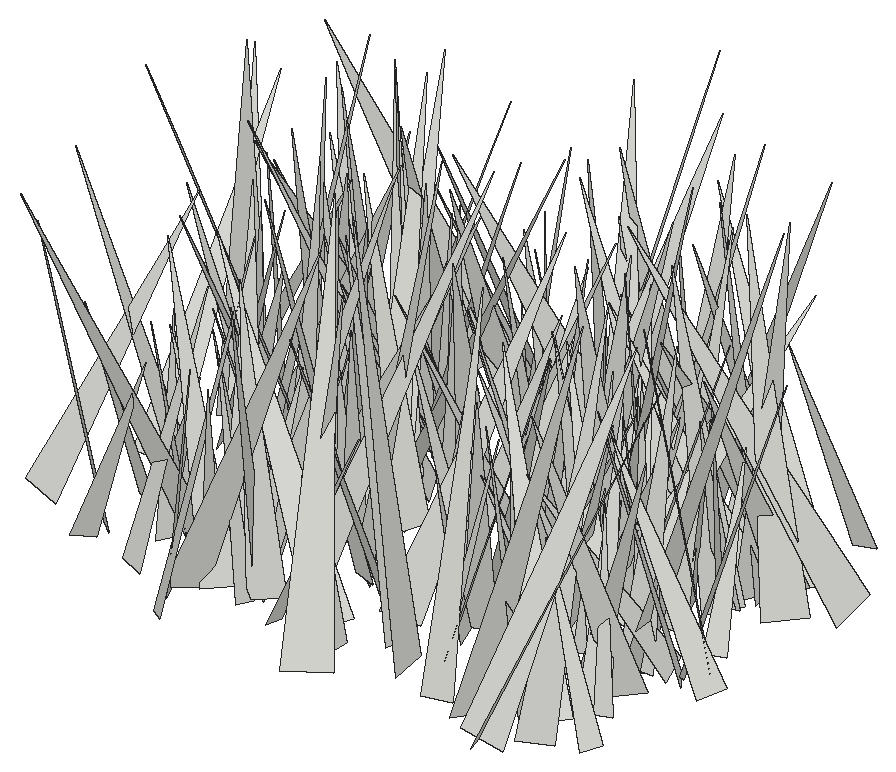
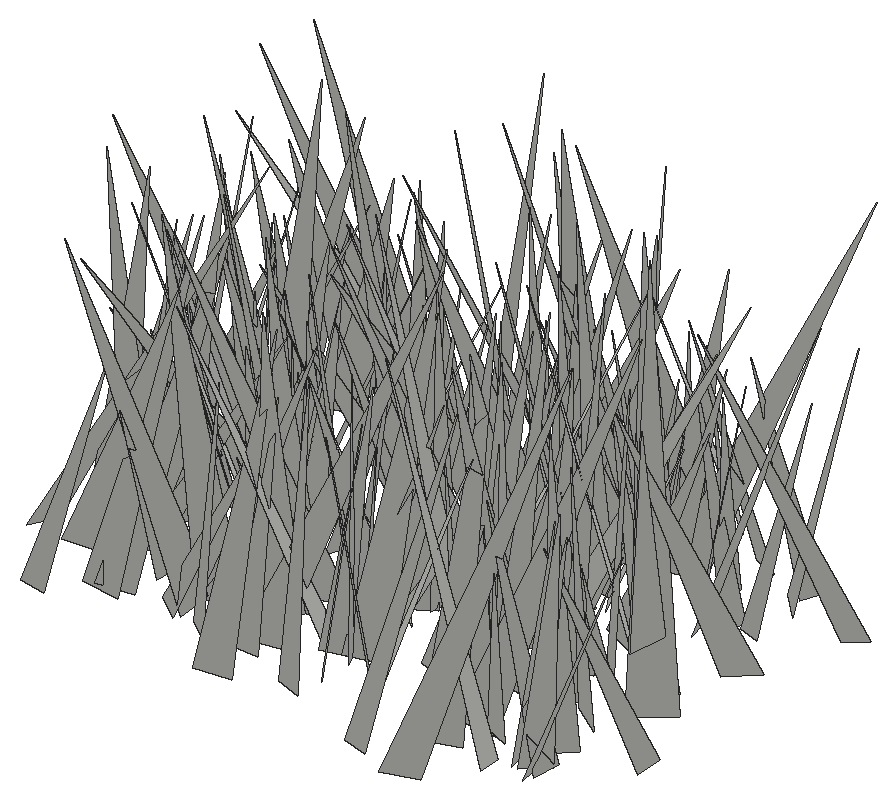
# SketchUp Ruby script. Lengths in inches.
U = 1.inch
M = Sketchup.active_model
def pt(a) = Geom::Point3d.new(a.map { |v| v * U })
def face(e, loops, mat)
  f = e.add_face(loops[0].map { |a| pt(a) })
  loops[1..].each { |l| e.add_face(l.map { |a| pt(a) }).erase! }
  f.material = f.back_material = mat if mat
  f
end
# faces: each face lists its corners as indices into pts; further lists are holes
def faces(e, pts, list, mat = nil) = list.each { |f| face(e, (f[0].is_a?(Array) ? f : [f]).map { |l| l.map { |i| pts[i] } }, mat) }
# xy, xz, yz: faces in a plane at the given z, y or x. An outline is a flat list of corners, or four numbers for a rectangle; further outlines are holes
def ring(l) = l.size == 4 ? [[l[0], l[1]], [l[2], l[1]], [l[2], l[3]], [l[0], l[3]]] : l.each_slice(2).to_a
def flat(e, list, mat, &to3) = list.each { |f| face(e, (f[0].is_a?(Array) ? f : [f]).map { |l| ring(l).map { |u, v| to3.(u, v) } }, mat) }
def xy(e, z, list, mat = nil) = flat(e, list, mat) { |x, y| [x, y, z] }
def xz(e, y, list, mat = nil) = flat(e, list, mat) { |x, z| [x, y, z] }
def yz(e, x, list, mat = nil) = flat(e, list, mat) { |y, z| [x, y, z] }
def lines(e, pts, list) = list.each { |a, b| e.add_line(pt(pts[a]), pt(pts[b])) }
# prism: a flat outline (further loops are holes) pulled along v
def prism(e, loops, v, mat = nil)
  f = face(e, loops, mat); d = Geom::Vector3d.new(v.map { |x| x * U })
  f.pushpull(f.normal.samedirection?(d) ? d.length : -d.length)
end
def box(e, o, s, mat = nil) = prism(e, [[o, [o[0] + s[0], o[1], o[2]], [o[0] + s[0], o[1] + s[1], o[2]], [o[0], o[1] + s[1], o[2]]]], [0, 0, s[2]], mat)
def at(x, y, z, deg = 0) = Geom::Transformation.translation(pt([x, y, z])) * Geom::Transformation.rotation(ORIGIN, Z_AXIS, deg.degrees)
def axes(o, x, y, z) = Geom::Transformation.new([*x, 0, *y, 0, *z, 0, *pt(o).to_a, 1])
def part(name) = M.definitions.add(name)
# library, detail: a bought-in or finely detailed component or shape, given as its bounding box
def library(name, o, s) = part(name).tap { |d| box(d.entities, o, s) }
def detail(e, o, s) = box(e.add_group.entities, o, s)
def put(e, d, t, mat = nil) = e.add_instance(d, t).tap { |i| i.material = mat if mat }
def group(e, t, mat = nil) = e.add_group.tap { |g| g.transformation = t; g.material = mat if mat }.entities
root = M.entities
c1 = part("fur_instance\#9")
p = [[0.8125,0,1.79],[0.67,-0.02,1.48],[0,-0.11,0],[0,0.11,0]]
faces(c1.entities,p,[[0,1,2,3]])
put(root,c1,axes([118.75,215.38,-27.1],[-3.28983,-1.54802,1.9149],[-2.00034,3.5437,-0.57187],[1.43591,1.38997,3.59058]))
put(root,c1,axes([118.43,218.14,-27.1],[-1.35129,-7.71927,0.81651],[-7.46816,1.06686,-2.27338],[-2.11671,1.16382,7.49966]))
put(root,c1,axes([125.51,216.04,-27.1],[-3.60239,-0.15597,0.87969],[-0.19043,3.7046,-0.12301],[0.87288,0.16452,3.60367]))
put(root,c1,axes([136.4,215.91,-27.1],[-3.21224,1.96871,0.46482],[2.01704,3.18335,0.45637],[0.15311,-0.63315,3.7398]))
put(root,c1,axes([120.625,217.96,-27.1],[5.99792,1.55177,2.60045],[2.40829,-5.94226,-2.00876],[-1.83589,-2.72525,5.86071]))
put(root,c1,axes([131.79,215.22,-27.1],[7.44072,-1.6859,2.03296],[-2.09272,-7.4711,1.46382],[-1.61112,1.91833,7.48758]))
put(root,c1,axes([133.125,214.13,-27.1],[-0.55252,7.61083,1.2014],[7.43516,0.84266,-1.91879],[2.02152,-1.01911,7.38568]))
put(root,c1,axes([134.1875,215.24,-27.1],[-5.16392,-1.1559,0.80889],[-1.35151,4.93357,-1.57791],[0.40477,1.72635,5.05098]))
put(root,c1,axes([125.68,214.08,-27.1],[-5.56313,6.05819,1.00831],[6.02083,5.64819,-0.71719],[1.2116,-0.25113,8.19364]))
put(root,c1,axes([114.08,216.65,-27.1],[3.45367,-2.54495,0.42724],[-2.57712,-3.36456,0.79082],[0.1334,0.88889,4.21654]))
put(root,c1,axes([123.74,216.53,-27.1],[6.28963,-0.96384,2.1084],[-1.07131,-6.61487,0.17192],[-2.05588,0.49827,6.36073]))
put(root,c1,axes([118.91,216.05,-27.1],[6.76451,-3.26106,1.25254],[-3.47694,-6.54929,1.72622],[-0.33809,2.1058,7.30844]))
put(root,c1,axes([128.125,216.47,-27.1],[-7.87878,-1.52664,2.20407],[-1.70967,8.13085,-0.47967],[2.06533,0.90687,8.01097]))
put(root,c1,axes([133.12,213.78,-27.1],[6.18332,3.30926,0.01495],[3.17233,-5.93637,1.96995],[-0.9422,1.73008,6.73082]))
put(root,c1,axes([122.71,216.04,-27.1],[3.9235,0.14114,0.37721],[0.06723,-3.8717,0.74932],[-0.3971,0.73898,3.85386]))
put(root,c1,axes([119.34,213.99,-27.1],[4.35483,5.04158,0.80125],[4.65214,-4.35304,2.10539],[-2.1017,0.81089,6.32055]))
put(root,c1,axes([118.79,217.6,-27.1],[3.85883,-1.0172,1.02296],[-0.87371,-3.97244,-0.65425],[-1.14794,-0.39587,3.93665]))
put(root,c1,axes([129.71,215.92,-27.1],[2.50571,3.8301,0.73521],[3.84486,-2.57244,0.29737],[-0.65369,-0.44905,4.56726]))
put(root,c1,axes([121.5625,217.11,-27.1],[-3.51075,4.42455,2.16586],[4.8357,3.60279,0.47842],[0.94002,-2.00904,5.62789]))
put(root,c1,axes([119.84,216.78,-27.1],[-3.34146,5.15286,1.47209],[5.35695,3.16362,1.08579],[-0.14849,-1.82317,6.0447]))
put(root,c1,axes([116.61,216.07,-27.1],[2.03381,4.83721,0.83738],[4.90479,-2.04045,-0.1258],[-0.20703,-0.82108,5.24587]))
put(root,c1,axes([121.15,216.45,-27.1],[-4.31173,0.11749,0.33288],[0.02447,4.16916,-1.1546],[0.35215,1.14887,4.15592]))
put(root,c1,axes([114.28,217.63,-27.1],[-4.01169,-3.78695,1.3287],[-4.00574,3.89344,-0.9976],[0.2459,1.64323,5.42581]))
put(root,c1,axes([125.25,219.08,-27.1],[-2.82637,-5.01502,0.69558],[-5.06125,2.81969,-0.23605],[0.13409,0.7222,5.75179]))
put(root,c1,axes([132.3,217.14,-27.1],[-3.8319,-0.08961,1.0116],[-0.27638,3.8917,-0.7022],[0.97723,0.7493,3.76807]))
put(root,c1,axes([134.18,216.58,-27.1],[-3.78417,5.30239,0.2634],[5.25954,3.70033,1.07214],[-0.72248,-0.83479,6.42541]))
put(root,c1,axes([124.35,217.11,-27.1],[-4.44973,5.42889,0.1833],[5.21151,4.19987,2.12315],[-1.53186,-1.48148,6.69068]))
put(root,c1,axes([135.0625,219.58,-27.1],[2.07945,-5.56592,1.40736],[-5.43571,-2.39045,-1.42237],[-1.84751,0.76846,5.76892]))
put(root,c1,axes([130.25,215.33,-27.1],[0.51601,7.02264,0.2402],[6.84431,-0.55684,1.57697],[-1.5908,-0.11784,6.86272]))
put(root,c1,axes([120.35,217.64,-27.1],[0.83525,-3.69964,2.10924],[-4.22949,-0.46947,0.8514],[0.49764,2.21949,3.69595]))
put(root,c1,axes([118.83,218.36,-27.1],[-2.76713,3.18046,1.2921],[3.43249,2.58898,0.97827],[0.05304,-1.61979,4.10065]))
put(root,c1,axes([134.68,215.03,-27.1],[-6.77077,3.15469,0.89527],[2.64884,6.47215,-2.77341],[1.93319,2.18084,6.93567]))
put(root,c1,axes([117.28,218.42,-27.1],[-3.57369,-1.9669,1.0397],[-2.0892,3.64317,-0.28897],[0.76478,0.76131,4.06896]))
put(root,c1,axes([128.33,219.27,-27.1],[-3.2792,-1.26365,1.37089],[-0.97388,3.52607,0.9207],[1.58988,-0.44645,3.3915]))
put(root,c1,axes([128.36,219.98,-27.1],[2.49567,-4.97649,0.70111],[-5.02561,-2.47346,0.33254],[-0.01412,0.77585,5.55727]))
put(root,c1,axes([120.59,217.56,-27.1],[4.03025,7.20792,1.49357],[7.34455,-3.82368,-1.36555],[0.49235,-1.96292,8.14446]))
put(root,c1,axes([126.84,217.54,-27.1],[-7.00273,-0.39667,0.95685],[-0.59042,6.90153,-1.45992],[0.85107,1.52402,6.86034]))
put(root,c1,axes([116.36,218.28,-27.1],[-3.76859,1.24193,1.36163],[1.17189,4.00702,-0.41131],[1.42236,-0.01087,3.94658]))
put(root,c1,axes([114.88,219.91,-27.1],[1.3305,-3.93215,0.09517],[-3.71952,-1.22514,1.38031],[1.27907,0.52755,3.91494]))
put(root,c1,axes([135.32,217.88,-27.1],[-0.19051,3.61425,0.52762],[3.57644,0.0773,0.76192],[-0.74175,-0.55561,3.53816]))
put(root,c1,axes([132.47,219.64,-27.1],[-4.25232,-1.15186,0.17503],[-1.13335,4.24309,0.38907],[0.27009,-0.33025,4.38835]))
put(root,c1,axes([114.16,219.99,-27.1],[-1.28236,-4.10189,0.60594],[-4.14572,1.27987,-0.10961],[0.07509,0.61118,4.29626]))
put(root,c1,axes([133.57,219.35,-27.1],[4.86131,-2.02952,0.59697],[-2.06386,-4.87843,0.22145],[-0.46454,0.43544,5.26329]))
put(root,c1,axes([119.67,218.16,-27.1],[-2.53684,6.34204,1.9532],[6.60869,2.60398,0.12835],[0.60133,-1.86275,6.82939]))
put(root,c1,axes([120.46,218.35,-27.1],[3.86814,-0.78573,1.02615],[-1.07279,-3.75781,1.16655],[-0.72076,1.37634,3.77081]))
put(root,c1,axes([135.16,221.83,-27.1],[-5.02387,-1.18033,0.42976],[-0.88594,4.58548,2.23734],[0.8905,-2.09699,4.65046]))
put(root,c1,axes([128.69,217.84,-27.1],[4.75922,3.00167,0.77273],[2.8511,-4.79497,1.06623],[-1.21588,0.50555,5.5248]))
put(root,c1,axes([128.02,220.89,-27.1],[6.9866,-0.46387,0.39437],[-0.38095,-6.874,-1.33651],[-0.47495,-1.31005,6.87325]))
put(root,c1,axes([111.05,218.15,-27.1],[0.65701,6.39206,0.99008],[6.12037,-0.29236,-2.17392],[2.09278,-1.15171,6.04683]))
put(root,c1,axes([134.65,218.26,-27.1],[-3.96377,3.38106,0.80717],[3.27975,4.04327,-0.83051],[1.15166,0.12228,5.14327]))
put(root,c1,axes([120.79,221.17,-27.1],[2.81621,-4.35059,0.38195],[-4.36621,-2.81499,0.12899],[-0.09891,0.39082,5.18093]))
put(root,c1,axes([123.21,220.25,-27.1],[-3.81075,-5.76969,1.72606],[-6.01138,3.52106,-1.50194],[-0.36316,2.25903,6.74947]))
put(root,c1,axes([115.74,220.55,-27.1],[-6.60705,-1.5953,0.55499],[-1.61141,6.62494,-0.14037],[0.50631,0.26714,6.79547]))
put(root,c1,axes([135.77,221.49,-27.1],[-4.16981,-3.31895,0.85743],[-3.36405,4.22145,-0.01946],[0.65859,0.54939,5.32938]))
put(root,c1,axes([122.56,217.82,-27.1],[3.274,7.7332,0.0389],[7.72076,-3.26624,-0.49451],[0.44025,-0.22856,8.38313]))
put(root,c1,axes([130.0625,219.08,-27.1],[4.92859,0.75105,0.39032],[0.57555,-4.66461,1.7081],[-0.62062,1.63853,4.68375]))
put(root,c1,axes([130.85,221.33,-27.1],[4.88822,-0.89007,0.63341],[-0.87396,-4.92864,-0.18113],[-0.65546,-0.06625,4.96529]))
put(root,c1,axes([137.24,221.32,-27.1],[-3.88127,2.88585,0.74535],[2.95869,3.58243,1.53633],[-0.36036,-1.66913,4.58608]))
put(root,c1,axes([117.11,221.5,-27.1],[-3.35519,-0.75879,1.11745],[-0.66434,3.53232,0.40387],[1.17606,-0.1694,3.41613]))
put(root,c1,axes([122.875,220.59,-27.1],[4.94057,6.27292,2.28459],[6.62263,-4.9638,-0.69253],[-0.84236,-2.23369,7.95482]))
put(root,c1,axes([121.28,222.14,-27.1],[4.3252,-1.84495,1.08949],[-1.74272,-4.45705,-0.62914],[-1.2465,-0.1704,4.65998]))
put(root,c1,axes([119.76,220.89,-27.1],[-1.17344,-6.36654,3.3674],[-7.15717,1.41187,0.17527],[0.80444,3.27459,6.4714]))
put(root,c1,axes([133.66,220.24,-27.1],[-3.54308,4.52564,0.44169],[4.5332,3.47169,0.79207],[-0.35583,-0.83417,5.69276]))
put(root,c1,axes([119.19,221.23,-27.1],[-3.56795,-1.90054,0.20659],[-1.88749,3.43261,-1.0196],[-0.30353,0.99505,3.91187]))
put(root,c1,axes([121.06,222.16,-27.1],[3.12862,-2.29976,0.97047],[-2.27,-3.26853,-0.42753],[-1.03819,0.21622,3.85932]))
put(root,c1,axes([119.6,222.34,-27.1],[-2.97,-5.19915,0.68344],[-5.09037,2.66981,-1.8109],[-1.25951,1.46972,5.70725]))
put(root,c1,axes([134.15,221.08,-27.1],[-0.55684,5.82392,2.02647],[6.12632,0.75415,-0.48394],[0.70204,-1.96161,5.83043]))
put(root,c1,axes([126.51,221.91,-27.1],[-4.66446,-0.17714,0.77084],[-0.14932,4.72517,0.1823],[0.77671,-0.15541,4.66426]))
put(root,c1,axes([135.9,222.8125,-27.1],[4.20893,3.73459,3.7879],[4.59902,-4.98198,-0.19834],[-2.67289,-2.69131,5.62342]))
put(root,c1,axes([131.53,223.89,-27.1],[4.41778,-6.32124,1.65754],[-6.32459,-4.6393,-0.83587],[-1.6447,0.86086,7.66656]))
put(root,c1,axes([124.6,222.95,-27.1],[3.18493,-3.37138,0.77047],[-3.44968,-3.17103,0.3845],[-0.24394,0.82581,4.62191]))
put(root,c1,axes([132.14,220.88,-27.1],[-4.57761,1.25738,1.06742],[0.91701,4.55759,-1.43608],[1.37093,1.14988,4.52473]))
put(root,c1,axes([131.1,222.18,-27.1],[1.65832,3.59632,1.35209],[3.82471,-1.68517,-0.20869],[-0.36513,-1.31848,3.95475]))
put(root,c1,axes([125.84,218.89,-27.1],[-5.17652,4.83446,1.05401],[3.91261,4.93311,-3.41105],[3.02894,1.88989,6.20751]))
put(root,c1,axes([118.93,224.83,-27.1],[7.2919,-1.58164,0.56037],[-1.39543,-7.10365,-1.89164],[-0.93186,-1.73896,7.21769]))
put(root,c1,axes([129.96,222.66,-27.1],[-5.05494,-2.22544,0.30278],[-2.23904,4.935,-1.10864],[-0.17591,1.1357,5.41072]))
put(root,c1,axes([127.45,224.33,-27.1],[-5.15654,-2.89646,0.02201],[-2.88562,5.14083,0.47427],[0.2514,-0.40276,5.89529]))
put(root,c1,axes([131.22,221.58,-27.1],[-1.86481,4.13252,0.34952],[4.14724,1.85655,0.17621],[-0.01744,-0.39104,4.53037]))
put(root,c1,axes([130.72,223.42,-27.1],[4.45339,-2.56263,0.11815],[-2.55046,-4.39735,0.75645],[0.27609,0.71411,5.08208]))
put(root,c1,axes([119.44,223.28,-27.1],[-6.03257,-5.76703,0.56772],[-5.59645,5.58532,-2.7307],[-1.50355,2.34912,7.8863]))
put(root,c1,axes([128.52,224.27,-27.1],[-4.47409,-0.55232,0.95951],[-0.288,4.43762,1.21151],[1.069,-1.11608,4.34221]))
put(root,c1,axes([119.45,222.77,-27.1],[5.54301,-4.89223,1.08245],[-4.92161,-5.01325,2.54471],[0.93987,2.60075,6.94141]))
put(root,c1,axes([132.03,224.33,-27.1],[-2.90046,-3.39812,1.38689],[-3.27993,3.19309,0.96417],[1.64705,0.37459,4.36237]))
put(root,c1,axes([133.33,222.43,-27.1],[-4.45117,0.87592,1.04433],[0.68712,4.52233,-0.86441],[1.17717,0.67238,4.45342]))
put(root,c1,axes([117.28,223.04,-27.1],[-0.49335,5.1966,1.87912],[5.02115,-0.36617,2.33091],[-2.30734,-1.90798,4.67065]))
put(root,c1,axes([134.33,220.7,-27.1],[7.79418,1.63756,2.08164],[0.8535,-7.67768,2.8441],[-2.50726,2.47704,7.43922]))
put(root,c1,axes([123.875,225.59,-27.1],[4.30968,-5.09044,0.61484],[-5.06109,-4.35201,-0.55619],[-0.82219,0.10671,6.64655]))
put(root,c1,axes([113.53,225.02,-27.1],[6.27835,0.76334,0.54412],[0.88551,-6.03847,-1.74618],[-0.30762,-1.80294,6.07875]))
put(root,c1,axes([116.91,225.69,-27.1],[-0.2881,-6.79413,1.19024],[-6.52945,0.65262,2.14482],[2.22333,1.03623,6.45314]))
put(root,c1,axes([130.15,224.71,-27.1],[-3.55733,-3.55392,1.20149],[-3.66341,3.64755,-0.05732],[0.80828,0.89081,5.02808]))
put(root,c1,axes([114.26,225.03,-27.1],[1.4923,-4.43759,0.64343],[-4.35505,-1.27294,1.3215],[1.06759,1.01025,4.49142]))
put(root,c1,axes([118.21,223.64,-27.1],[3.92442,2.27765,0.90763],[2.32456,-4.0011,-0.01041],[-0.77966,-0.46478,4.53747]))
put(root,c1,axes([129.31,224.72,-27.1],[1.81609,-4.28388,1.69446],[-4.45246,-2.09973,-0.53642],[-1.18256,1.32684,4.62191]))
put(root,c1,axes([131.38,222.68,-27.1],[7.46967,2.68884,2.29218],[2.3982,-7.79505,1.32883],[-2.59473,0.53597,7.82688]))
put(root,c1,axes([124.96,223.64,-27.1],[0.90877,4.85728,1.17196],[4.86719,-0.59112,-1.32422],[1.13009,-1.36012,4.76083]))
put(root,c1,axes([122.35,223.92,-27.1],[-5.92125,2.00992,1.02968],[2.02644,6.00419,-0.06686],[0.99676,-0.26678,6.25272]))
put(root,c1,axes([135.64,223.44,-27.1],[-2.23531,2.8422,0.49749],[2.78374,2.28983,-0.57415],[0.75919,-0.0278,3.57002]))
put(root,c1,axes([135.74,221.55,-27.1],[4.27823,3.00126,0.70858],[2.21616,-3.83495,2.86263],[-2.14435,2.02448,4.3722]))
put(root,c1,axes([131.73,224,-27.1],[5.13146,2.31605,0.71954],[2.33013,-5.17519,0.0403],[-0.67253,-0.25897,5.62978]))
put(root,c1,axes([121.19,226.44,-27.1],[-6.73685,-3.71008,0.0403],[-3.70619,6.73292,0.28887],[0.17463,-0.23362,7.68547]))
put(root,c1,axes([123.37,224.71,-27.1],[5.69837,-0.41307,2.53776],[-0.52377,-6.22748,0.16244],[-2.51724,0.36068,5.71101]))
put(root,c1,axes([133.03,225.4,-27.1],[4.02483,1.17033,1.17041],[1.40502,-4.04247,-0.78939],[-0.87491,-1.10794,4.11653]))
put(root,c1,axes([134.375,225.34,-27.1],[-3.74193,-1.93414,1.83822],[-1.95383,4.14237,0.38123],[1.81727,0.47108,4.19495]))
put(root,c1,axes([131.4,224.875,-27.1],[1.02394,3.35387,1.44831],[3.57422,-1.23084,0.32333],[-0.75567,-1.27715,3.49176]))
put(root,c1,axes([112.5625,222.32,-27.1],[-2.48989,6.58556,0.19317],[6.42005,2.47161,-1.51018],[1.47984,0.3578,6.87667]))
put(root,c1,axes([113.17,226.39,-27.1],[4.71718,-6.41333,2.08506],[-6.64537,-4.85367,0.10513],[-1.14777,1.74389,7.96063]))
put(root,c1,axes([113.81,226.07,-27.1],[4.65785,-0.69082,1.21899],[-0.53967,-4.78978,-0.65231],[-1.29303,-0.48941,4.6634]))
put(root,c1,axes([133.98,225.98,-27.1],[4.51203,-4.20905,2.90182],[-4.30887,-5.21386,-0.8628],[-2.75143,1.26279,6.10984]))
put(root,c1,axes([119.36,226.25,-27.1],[-4.57691,0.82768,1.57562],[1.18388,4.66198,0.99001],[1.32893,-1.30255,4.54457]))
put(root,c1,axes([115.57,225.69,-27.1],[-3.42106,-4.15596,2.05732],[-4.44833,3.66341,0.00339],[1.31032,1.58608,5.3829]))
put(root,c1,axes([133.96,226.26,-27.1],[0.76269,-3.95415,0.89534],[-4.04548,-0.80213,-0.09639],[-0.26648,0.86018,4.02588]))
put(root,c1,axes([114.61,226.61,-27.1],[5.46808,5.3055,1.78388],[5.41419,-4.38056,-3.56761],[1.42026,-3.72732,6.73205]))
put(root,c1,axes([116.31,223.43,-27.1],[-5.10797,-4.03263,5.02727],[-5.71036,5.80586,-1.14484],[2.98787,4.202,6.40647]))
put(root,c1,axes([126.93,225.28,-27.1],[3.29579,4.51514,1.8086],[4.80118,-3.36974,-0.33663],[-0.7786,-1.66678,5.57991]))
put(root,c1,axes([115.91,227.55,-27.1],[6.82649,-0.20783,2.36031],[0.47416,-6.93274,-1.9818],[-2.32152,-2.02711,6.5358]))
put(root,c1,axes([129.52,224.95,-27.1],[-4.01098,-1.65554,1.8183],[-2.11594,4.09606,-0.93811],[1.25294,1.61753,4.23659]))
put(root,c1,axes([117.26,226.63,-27.1],[4.37094,-3.26497,1.75227],[-3.26747,-4.6741,-0.55863],[-1.74761,0.57306,5.42707]))
put(root,c1,axes([119.2,228.13,-27.1],[1.9027,-5.40071,0.1352],[-5.35593,-1.9045,-0.70218],[-0.70705,-0.10684,5.68285]))
put(root,c1,axes([134.92,228.47,-27.1],[3.41213,-4.67618,0.33772],[-4.46229,-3.36731,-1.54031],[-1.43828,-0.64649,5.58003]))
put(root,c1,axes([129.73,227.15,-27.1],[4.8829,2.83209,2.83107],[3.60518,-5.05239,-1.16384],[-1.7431,-2.51617,5.52349]))
put(root,c1,axes([119.6,228.6,-27.1],[-3.6044,-3.37024,0.34721],[-3.01204,3.4196,1.92476],[1.55135,-1.19103,4.54373]))
put(root,c1,axes([120.65,225.08,-27.1],[7.61599,0.93725,0.32253],[0.89381,-7.57423,0.90437],[-0.42844,0.85927,7.61996]))
put(root,c1,axes([131.21,223.36,-27.1],[-1.51427,6.54379,0.36236],[5.84338,1.51647,-2.96661],[2.96773,0.35306,6.02606]))
put(root,c1,axes([133.4,223.9,-27.1],[1.19903,6.87384,0.5978],[6.78552,-1.2847,1.16229],[-1.25048,-0.38022,6.88014]))
put(root,c1,axes([121.6,223.21,-27.1],[-6.67493,4.02137,0.12146],[3.83511,6.43107,-2.16198],[1.21576,1.79188,7.48679]))
put(root,c1,axes([127.54,227.09,-27.1],[3.13574,-5.33007,1.5739],[-5.55752,-3.01682,0.85589],[-0.02918,1.79133,6.12454]))
put(root,c1,axes([118.34,227.78,-27.1],[-1.31696,-6.51866,1.83434],[-6.75362,1.40125,0.13086],[0.49623,1.77078,6.64907]))
put(root,c1,axes([137.375,228.71,-27.1],[-8.16776,0.06376,0.0825],[0.08376,7.86119,2.21763],[0.06209,-2.2183,7.8612]))
put(root,c1,axes([130.9,224.99,-27.1],[-2.1836,4.82414,0.14178],[4.82373,2.17653,0.23433],[-0.15514,-0.2257,5.29014]))
put(root,c1,axes([123.6875,227.08,-27.1],[-2.7685,-2.84273,0.0732],[-2.6967,2.59213,-1.32656],[-0.90237,0.97511,3.73978]))
put(root,c1,axes([123.1,229.34,-27.1],[2.89826,-6.60565,0.55734],[-6.55377,-2.94663,-0.84295],[-0.99662,0.16719,7.16407]))
put(root,c1,axes([125.18,227.44,-27.1],[4.42222,0.57042,2.59632],[0.96066,-5.04183,-0.52855],[-2.47858,-0.93641,4.42741]))
put(root,c1,axes([119.11,228.56,-27.1],[8.07507,1.50255,0.4439],[1.56674,-7.73574,-2.31627],[0.00564,-2.35841,7.88031]))
put(root,c1,axes([123.63,226.22,-27.1],[4.56915,3.9518,0.34933],[3.96081,-4.51383,-0.74378],[0.22516,-0.79028,5.99505]))
put(root,c1,axes([135.98,226.81,-27.1],[-4.89648,5.17695,2.06152],[5.4889,4.95404,0.59637],[0.96057,-1.91907,7.10075]))
put(root,c1,axes([125.12,225.94,-27.1],[-0.69382,4.82103,0.91338],[4.82167,0.84094,-0.77604],[0.90996,-0.78004,4.80848]))
put(root,c1,axes([114.05,225.41,-27.1],[-5.08982,4.44528,0.70369],[4.40622,5.13821,-0.58816],[0.91699,-0.01575,6.73207]))
put(root,c1,axes([132.63,230.78,-27.1],[4.86562,-4.5964,0.06859],[-4.19123,-4.47675,-2.68294],[-1.88818,-1.90726,6.13213]))
put(root,c1,axes([124.48,228.01,-27.1],[-4.64353,0.24048,0.81476],[0.40253,4.60984,0.93348],[0.74809,-0.98772,4.55508]))
put(root,c1,axes([117.37,230.66,-27.1],[2.70234,-6.75975,0.1599],[-6.39067,-2.60962,-2.31767],[-2.20886,-0.71979,6.90111]))
put(root,c1,axes([121.1875,224.99,-27.1],[-7.30125,2.0292,0.54339],[1.84392,7.1322,-1.85816],[1.00641,1.65384,7.34664]))
put(root,c1,axes([126.63,228.12,-27.1],[3.82304,5.79974,2.60132],[6.29108,-3.01834,-2.51622],[0.9089,-3.50316,6.47466]))
put(root,c1,axes([133.48,228.09,-27.1],[-5.14523,1.96025,0.06602],[1.88898,4.90265,1.64806],[-0.52792,-1.56261,5.25356]))
put(root,c1,axes([134.15,227.36,-27.1],[6.73151,-1.98165,2.55494],[-2.23492,-7.11595,0.36912],[-2.33662,1.09735,7.00742]))
put(root,c1,axes([119.16,228.23,-27.1],[5.28351,-1.61661,1.62366],[-1.56193,-5.52709,-0.42043],[-1.67632,0.05465,5.50927]))
put(root,c1,axes([120.97,228.52,-27.1],[-0.75955,-3.70224,0.74684],[-3.72635,0.61048,-0.76351],[-0.61539,0.87293,3.70143]))
put(root,c1,axes([125.07,226.8,-27.1],[-3.90269,-1.36809,1.23152],[-1.73858,3.68797,-1.41263],[0.60468,1.77384,3.88679]))
put(root,c1,axes([119.1,227.6,-27.1],[4.24793,5.0228,3.04998],[5.34423,-4.86703,0.57187],[-2.44337,-1.91294,6.55335]))
put(root,c1,axes([120.46,224.95,-27.1],[-0.64935,7.68845,0.01437],[7.6155,0.6412,1.06165],[-1.05669,-0.10353,7.64243]))
put(root,c1,axes([134.51,227.54,-27.1],[-6.69372,-1.63538,1.73187],[-1.91789,6.76382,-1.02573],[1.41263,1.43387,6.81383]))
put(root,c1,axes([126.54,230.65,-27.1],[-6.66712,2.68909,2.42043],[3.53397,5.92752,3.14894],[0.77508,-3.89533,6.46266]))
put(root,c1,axes([130.28,225.76,-27.1],[5.47327,5.90798,0.9862],[5.7796,-5.55993,1.23167],[-1.57262,0.12835,7.95889]))
put(root,c1,axes([128.42,228.16,-27.1],[4.16572,3.95636,0.93283],[4.06431,-4.03236,-1.04767],[0.06588,-1.40123,5.64875]))
put(root,c1,axes([120.16,228,-27.1],[1.76175,3.91399,1.38102],[4.01071,-1.99148,0.5277],[-1.06803,-1.02224,4.25965]))
put(root,c1,axes([113.99,230.21,-27.1],[4.00821,-3.73033,0.31245],[-3.73197,-4.01777,-0.09299],[-0.29215,0.14465,5.47471]))
put(root,c1,axes([124.15,229.62,-27.1],[1.70929,-4.46495,1.67991],[-4.63149,-1.98085,-0.55231],[-1.1433,1.34907,4.74893]))
put(root,c1,axes([132.97,231.14,-27.1],[-0.03159,-6.8611,0.78211],[-6.88005,-0.03586,-0.59249],[-0.59273,0.78192,6.83555]))
put(root,c1,axes([114.78,227.91,-27.1],[2.34142,5.16985,1.64131],[5.10687,-2.70355,1.23051],[-1.82787,-0.93109,5.54034]))
put(root,c1,axes([126.36,226.97,-27.1],[0.38295,8.08113,1.09098],[7.9956,-0.1576,-1.6392],[1.60161,-1.14545,7.92239]))
put(root,c1,axes([123.53,229.48,-27.1],[-4.21315,-2.34987,2.26772],[-2.4638,4.71684,0.31027],[2.14339,0.80291,4.81418]))
put(root,c1,axes([129.85,228.73,-27.1],[-6.207,1.9177,0.03314],[1.91765,6.20287,0.22937],[-0.03607,-0.22893,6.49244]))
put(root,c1,axes([117.54,232.24,-27.1],[2.10072,-7.09935,0.00934],[-7.09522,-2.09917,0.25546],[0.24231,0.08144,7.39923]))
put(root,c1,axes([129.44,229.17,-27.1],[3.63637,-5.76719,3.12725],[-6.51934,-3.57646,0.98508],[-0.73369,3.19558,6.74635]))
put(root,c1,axes([111.13,229.14,-27.1],[4.26787,-0.90452,0.30078],[-0.95208,-4.11231,1.14272],[-0.04649,1.18073,4.21035]))
put(root,c1,axes([130.48,230.65,-27.1],[-2.43952,-3.83837,0.4143],[-3.75379,2.24378,-1.31547],[-0.90209,1.04325,4.3536]))
put(root,c1,axes([123.49,231.14,-27.1],[-3.34648,-2.86729,1.25208],[-2.75468,3.56945,0.81158],[1.4835,0.16004,4.33146]))
put(root,c1,axes([135.27,229.14,-27.1],[-3.78872,6.01371,0.63065],[5.87535,3.48538,2.06137],[-1.42923,-1.61377,6.8022]))
put(root,c1,axes([131.91,228.82,-27.1],[-3.54385,2.2292,0.7922],[1.93522,3.55225,-1.33876],[1.36083,0.75365,3.96686]))
put(root,c1,axes([127.14,228.85,-27.1],[-5.31707,5.30249,0.96243],[5.27581,5.39738,-0.58989],[1.09932,-0.2564,7.48596]))
put(root,c1,axes([113.87,232.18,-27.1],[-4.07009,-1.55263,0.42821],[-1.43545,4.0247,0.94922],[0.73043,-0.7422,4.25151]))
put(root,c1,axes([114.78,230.92,-27.1],[-3.50037,2.65675,1.28484],[2.86731,3.53339,0.50538],[0.69832,-1.19104,4.36526]))
put(root,c1,axes([129.83,229.89,-27.1],[7.1879,-0.3196,1.18159],[-0.53762,-7.14753,1.33717],[-1.09967,1.40532,7.06966]))
put(root,c1,axes([126.66,231.39,-27.1],[0.55696,-4.64877,2.01019],[-4.98122,-0.86859,-0.62855],[-0.91614,1.89648,4.63963]))
put(root,c1,axes([134.92,232.37,-27.1],[0.09538,-4.31944,0.7575],[-4.29634,-0.24392,-0.84995],[-0.8791,0.72346,4.23607]))
put(root,c1,axes([128.7,231.26,-27.1],[2.49829,3.83803,2.30798],[4.11646,-3.0089,0.54773],[-1.76409,-1.58579,4.54664]))
put(root,c1,axes([115.36,232.375,-27.1],[6.89965,2.05968,0.48381],[2.11498,-6.67017,-1.76557],[0.05673,-1.82978,6.98071]))
put(root,c1,axes([113.62,231.5,-27.1],[4.85484,-0.93426,0.93937],[-1.01134,-4.91828,0.33525],[-0.85583,0.51221,4.93253]))
put(root,c1,axes([116.41,230.68,-27.1],[0.5097,3.85536,0.87755],[3.83119,-0.70034,0.85159],[-0.9777,-0.73445,3.79452]))
put(root,c1,axes([114.83,231.34,-27.1],[-5.03296,-0.41167,1.23228],[-0.52474,5.15421,-0.42127],[1.18855,0.5323,5.03216]))
put(root,c1,axes([119.65,234.19,-27.1],[-2.17037,-5.72704,0.1674],[-5.69455,2.17595,0.61228],[0.63178,-0.0613,6.09382]))
put(root,c1,axes([125.42,228.57,-27.1],[6.25178,5.32919,0.93445],[4.93149,-6.20008,2.36594],[-2.22574,1.23164,7.86685]))
put(root,c1,axes([119.88,233.78,-27.1],[-3.92471,-3.72483,0.22437],[-3.66233,3.90735,0.80501],[0.71557,-0.43166,5.35067]))
put(root,c1,axes([114.01,231.56,-27.1],[3.17127,-3.30736,3.04126],[-3.82504,-3.9403,-0.2965],[-2.35731,1.94429,4.57249]))
put(root,c1,axes([121.37,231.06,-27.1],[3.52114,3.87417,1.40413],[3.91467,-3.72163,0.45161],[-1.28689,-0.72073,5.21571]))
put(root,c1,axes([123.875,232.47,-27.1],[-1.84582,-5.09705,1.94608],[-5.40108,1.99766,0.10933],[0.77171,1.78987,5.41987]))
put(root,c1,axes([117.24,234.8,-27.1],[-7.12654,1.94071,2.81889],[3.04033,6.57978,3.15641],[1.57127,-3.9294,6.67765]))
put(root,c1,axes([126.48,233.27,-27.1],[1.47343,-6.07806,1.78682],[-6.21699,-1.74005,-0.79238],[-1.21846,1.52838,6.20371]))
